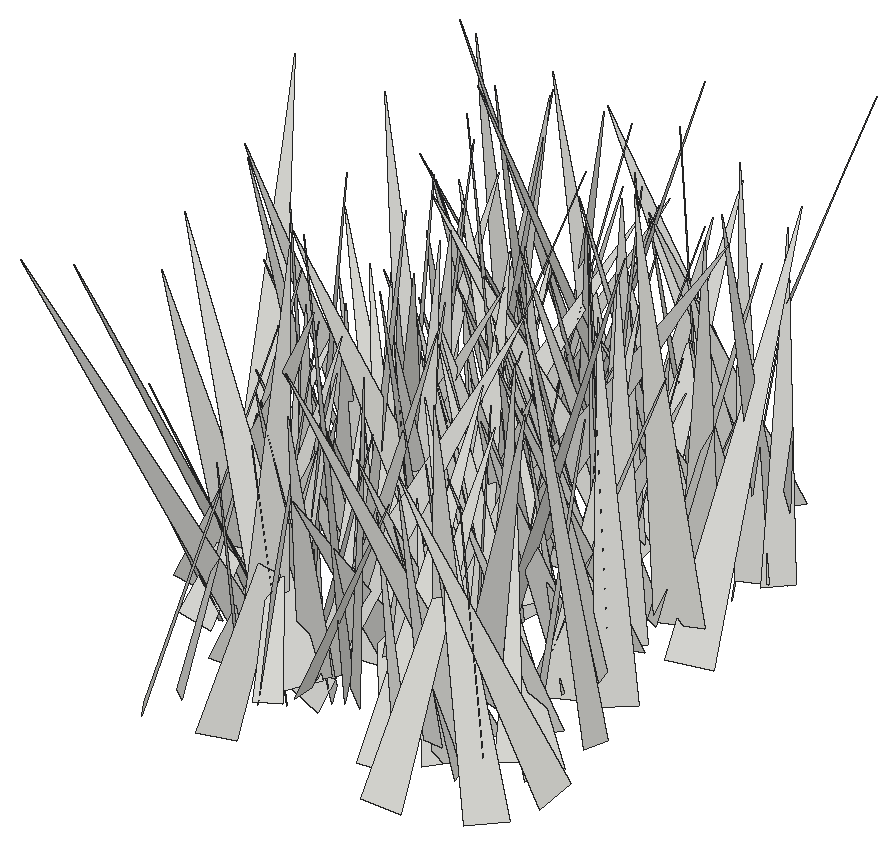
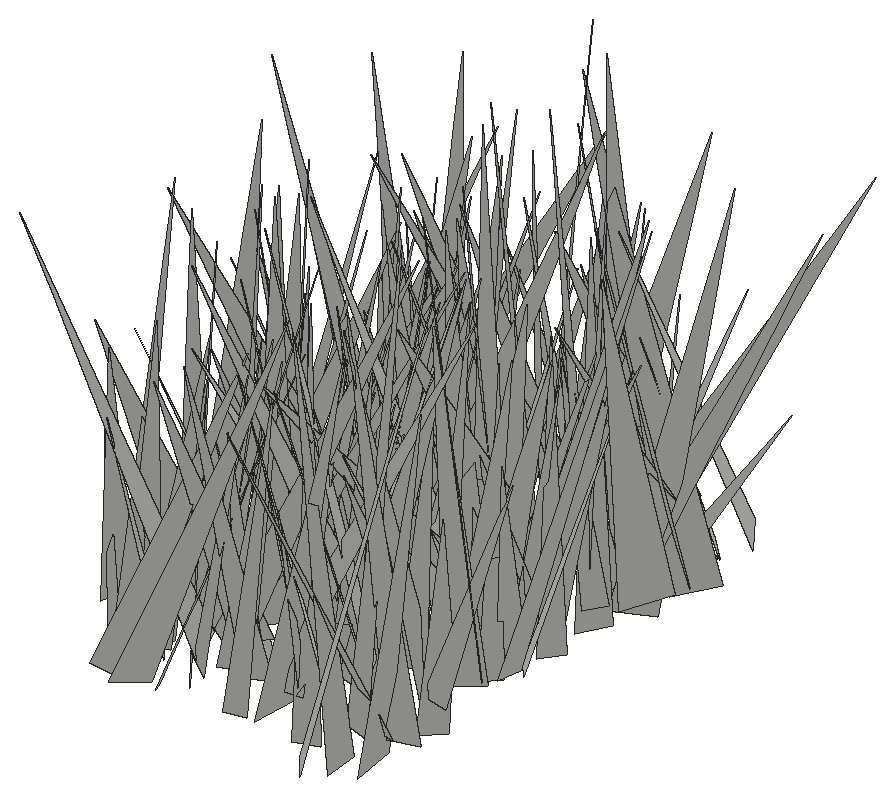
# SketchUp Ruby script. Lengths in inches.
U = 1.inch
M = Sketchup.active_model
def pt(a) = Geom::Point3d.new(a.map { |v| v * U })
def face(e, loops, mat)
  f = e.add_face(loops[0].map { |a| pt(a) })
  loops[1..].each { |l| e.add_face(l.map { |a| pt(a) }).erase! }
  f.material = f.back_material = mat if mat
  f
end
# faces: each face lists its corners as indices into pts; further lists are holes
def faces(e, pts, list, mat = nil) = list.each { |f| face(e, (f[0].is_a?(Array) ? f : [f]).map { |l| l.map { |i| pts[i] } }, mat) }
# xy, xz, yz: faces in a plane at the given z, y or x. An outline is a flat list of corners, or four numbers for a rectangle; further outlines are holes
def ring(l) = l.size == 4 ? [[l[0], l[1]], [l[2], l[1]], [l[2], l[3]], [l[0], l[3]]] : l.each_slice(2).to_a
def flat(e, list, mat, &to3) = list.each { |f| face(e, (f[0].is_a?(Array) ? f : [f]).map { |l| ring(l).map { |u, v| to3.(u, v) } }, mat) }
def xy(e, z, list, mat = nil) = flat(e, list, mat) { |x, y| [x, y, z] }
def xz(e, y, list, mat = nil) = flat(e, list, mat) { |x, z| [x, y, z] }
def yz(e, x, list, mat = nil) = flat(e, list, mat) { |y, z| [x, y, z] }
def lines(e, pts, list) = list.each { |a, b| e.add_line(pt(pts[a]), pt(pts[b])) }
# prism: a flat outline (further loops are holes) pulled along v
def prism(e, loops, v, mat = nil)
  f = face(e, loops, mat); d = Geom::Vector3d.new(v.map { |x| x * U })
  f.pushpull(f.normal.samedirection?(d) ? d.length : -d.length)
end
def box(e, o, s, mat = nil) = prism(e, [[o, [o[0] + s[0], o[1], o[2]], [o[0] + s[0], o[1] + s[1], o[2]], [o[0], o[1] + s[1], o[2]]]], [0, 0, s[2]], mat)
def at(x, y, z, deg = 0) = Geom::Transformation.translation(pt([x, y, z])) * Geom::Transformation.rotation(ORIGIN, Z_AXIS, deg.degrees)
def axes(o, x, y, z) = Geom::Transformation.new([*x, 0, *y, 0, *z, 0, *pt(o).to_a, 1])
def part(name) = M.definitions.add(name)
# library, detail: a bought-in or finely detailed component or shape, given as its bounding box
def library(name, o, s) = part(name).tap { |d| box(d.entities, o, s) }
def detail(e, o, s) = box(e.add_group.entities, o, s)
def put(e, d, t, mat = nil) = e.add_instance(d, t).tap { |i| i.material = mat if mat }
def group(e, t, mat = nil) = e.add_group.tap { |g| g.transformation = t; g.material = mat if mat }.entities
root = M.entities
c1 = part("fur_instance\#9")
p = [[0.8125,0,1.79],[0.67,-0.02,1.48],[0,-0.11,0],[0,0.11,0]]
faces(c1.entities,p,[[0,1,2,3]])
put(root,c1,axes([65.37,132.02,-27.1],[-6.50457,4.89284,0.5628],[4.72218,6.46057,-1.59001],[1.39918,0.94188,7.98255]))
put(root,c1,axes([66.375,129.34,-27.1],[-2.80536,-2.90649,0.0794],[-2.63209,2.49174,-1.78533],[-1.23535,1.29136,3.62358]))
put(root,c1,axes([67.03,130.54,-27.1],[-2.83632,-6.0499,0.28173],[-5.90232,2.69141,-1.62612],[-1.35766,0.93829,6.48088]))
put(root,c1,axes([65.68,137.62,-27.1],[-3.97352,-3.33663,0.47318],[-3.25036,3.98768,0.8243],[0.89005,-0.33346,5.12275]))
put(root,c1,axes([65.8125,138.13,-27.1],[-7.05336,-2.15617,1.71578],[-1.62887,7.06566,2.18314],[2.22256,-1.66441,7.04506]))
put(root,c1,axes([66.8,143.5,-28.22],[-7.05246,-0.20222,1.59365],[-0.38202,7.18084,-0.77939],[1.56034,0.84409,7.01218]))
put(root,c1,axes([68.76,129.2,-28.22],[-1.39061,-8.04384,0.83594],[-7.45661,0.94696,-3.29214],[-3.13068,1.31752,7.46987]))
put(root,c1,axes([66.67,136.97,-27.1],[-4.24883,1.88722,0.42776],[1.75815,4.19597,-1.04876],[0.80838,0.79335,4.52927]))
put(root,c1,axes([66.56,140.84,-27.1],[-0.08918,-3.86635,0.81214],[-3.84672,-0.10019,-0.89937],[-0.90053,0.81086,3.76135]))
put(root,c1,axes([66.54,131.21,-28.22],[4.91943,-4.73173,2.30235],[-4.40019,-5.42749,-1.75256],[-2.8859,0.2095,6.59686]))
put(root,c1,axes([68.17,136.98,-27.1],[-6.64184,2.29308,0.28161],[2.23011,6.58737,-1.04152],[0.60342,0.8944,6.94892]))
put(root,c1,axes([66.06,136.18,-27.1],[1.11267,-4.69864,0.20362],[-4.67497,-1.12782,-0.47895],[-0.51316,0.0867,4.80478]))
put(root,c1,axes([67.26,146.49,-27.1],[-6.10704,-5.17922,1.29191],[-4.99805,6.23748,1.37932],[1.87424,-0.24245,7.88782]))
put(root,c1,axes([67.74,130.69,-28.22],[-3.26059,-4.43586,0.10579],[-4.43536,3.26207,0.0775],[0.12511,0.03932,5.50476]))
put(root,c1,axes([65.54,136.41,-27.1],[4.72712,-1.54603,0.79765],[-1.39638,-4.74943,-0.93014],[-1.03759,-0.65178,4.88576]))
put(root,c1,axes([65.35,130.17,-27.1],[3.97347,4.57155,1.31094],[4.73936,-3.94824,-0.59665],[-0.39506,-1.38509,6.02757]))
put(root,c1,axes([68.65,133.42,-28.22],[-2.69995,-7.06667,2.40673],[-7.39529,2.18224,-1.88876],[-1.01973,2.88442,7.32531]))
put(root,c1,axes([65.8,128.78,-27.1],[-0.63862,5.35473,0.03552],[5.1577,0.62471,-1.44573],[1.43964,0.13724,5.19527]))
put(root,c1,axes([68.1875,134.67,-28.22],[-5.31115,0.249,1.00047],[0.14264,5.37711,-0.58108],[1.02108,0.54405,5.28514]))
put(root,c1,axes([67.35,132.58,-27.1],[-4.34525,-4.69158,2.51984],[-5.05188,4.66036,-0.03462],[1.68493,1.87398,6.3946]))
put(root,c1,axes([66.07,138.71,-27.1],[4.73789,-1.18845,0.72275],[-0.9672,-4.65874,-1.32025],[-0.99966,-1.12521,4.70287]))
put(root,c1,axes([69.15,134.625,-27.1],[-3.00084,5.06154,0.45444],[5.0055,2.85272,1.2797],[-0.87785,-1.03611,5.74339]))
put(root,c1,axes([65.71,143.39,-27.1],[-0.42435,-6.57592,2.54627],[-6.78158,1.0798,1.65847],[1.93298,2.34469,6.37748]))
put(root,c1,axes([67.03,126.5,-28.22],[3.04107,3.48011,0.59696],[3.3547,-3.09349,0.94446],[-1.10161,0.1866,4.52408]))
put(root,c1,axes([66.43,139.42,-27.1],[2.75053,-5.09352,1.52718],[-5.31748,-2.64324,0.76119],[-0.02665,1.70616,5.73847]))
put(root,c1,axes([68.98,133.01,-27.1],[-0.44719,-4.16584,0.88919],[-4.01944,0.11666,-1.47491],[-1.41032,0.98845,3.92158]))
put(root,c1,axes([66.71,125.11,-28.22],[5.18703,3.91751,0.7095],[3.72248,-5.18551,1.41748],[-1.41191,0.72053,6.34373]))
put(root,c1,axes([66.6,140.875,-28.22],[6.40589,-1.32849,1.4611],[-0.83624,-6.31798,-2.07823],[-1.78897,-1.80373,6.20333]))
put(root,c1,axes([66.84,132.75,-28.22],[5.79339,-2.08626,1.56673],[-1.97661,-6.00002,-0.68061],[-1.70297,-0.13319,6.11985]))
put(root,c1,axes([66.38,133.23,-27.1],[3.1539,-2.32332,0.00557],[-2.32207,-3.15188,0.13648],[0.07647,0.11319,3.91488]))
put(root,c1,axes([68.6,134.68,-27.1],[-1.93771,-4.14246,0.35212],[-4.15628,1.93921,-0.05843],[0.0961,0.34375,4.57288]))
put(root,c1,axes([67.24,143.76,-27.1],[-3.46246,-6.72611,1.90114],[-6.59046,3.84836,1.61233],[2.32826,0.89059,7.39118]))
put(root,c1,axes([67.82,130.51,-28.22],[0.58745,4.61701,1.14714],[4.75417,-0.52722,-0.31264],[0.17496,-1.17604,4.64372]))
put(root,c1,axes([70.76,127.48,-27.1],[-6.11884,4.72961,1.11538],[4.85918,5.97068,1.339],[0.0418,-1.7422,7.61686]))
put(root,c1,axes([68.25,138.9375,-28.22],[6.51752,3.06728,2.32468],[2.5593,-6.86862,1.88745],[-2.87443,0.8392,6.95153]))
put(root,c1,axes([68.92,128.92,-27.1],[-4.7564,-0.43454,1.78324],[-0.95829,4.81251,-1.3833],[1.56539,1.62573,4.5715]))
put(root,c1,axes([64.67,130.49,-27.1],[3.10816,-7.62871,0.22312],[-7.12075,-2.81203,3.04879],[2.74626,1.34273,7.65263]))
put(root,c1,axes([68.53,127.69,-28.22],[-2.76326,-3.0585,1.38467],[-3.15346,2.97986,0.28892],[1.15213,0.82059,4.11176]))
put(root,c1,axes([67.52,132.16,-27.1],[6.90611,3.10223,2.59996],[3.46907,-7.18559,-0.64093],[-2.08547,-1.6797,7.5437]))
put(root,c1,axes([67.55,144.13,-28.22],[6.8953,0.9557,1.85973],[1.13553,-7.09282,-0.56526],[-1.75571,-0.83402,6.93822]))
put(root,c1,axes([68.43,139.6,-27.1],[3.6116,-2.54944,1.03868],[-2.46348,-3.75778,-0.65768],[-1.22872,0.0404,4.37159]))
put(root,c1,axes([67.95,136.85,-28.22],[5.70767,4.90783,2.44546],[5.23724,-5.92496,-0.33273],[-1.62433,-1.85811,7.52021]))
put(root,c1,axes([68.91,138.86,-27.1],[-2.94733,3.27814,0.42411],[3.06608,2.92358,-1.29021],[1.23501,0.56503,4.21525]))
put(root,c1,axes([66.34,143.4,-27.1],[3.26284,4.45559,0.15103],[4.26787,-3.06768,-1.7017],[1.28856,-1.1217,5.25381]))
put(root,c1,axes([69.94,128.25,-27.1],[0.78619,5.10987,0.99795],[4.99569,-1.02461,1.31074],[-1.46621,-0.75112,5.00108]))
put(root,c1,axes([69.73,130.56,-28.22],[-3.33951,2.40161,0.05247],[2.31618,3.24301,-1.02031],[0.63702,0.79874,3.98485]))
put(root,c1,axes([66.95,128.88,-28.22],[2.87453,-4.20489,0.68169],[-4.14129,-2.56592,1.63539],[0.99777,1.46412,4.82385]))
put(root,c1,axes([71.49,142.23,-27.1],[-3.69679,-5.87263,0.02895],[-5.78236,3.6339,-1.23044],[-1.02613,0.67962,6.82936]))
put(root,c1,axes([69.74,131.6,-28.22],[-6.65412,4.03174,0.74119],[3.28122,6.08544,-3.64454],[2.45722,2.79179,6.87384]))
put(root,c1,axes([70.47,139.96,-28.22],[-0.74223,-7.02206,1.66779],[-7.14663,0.48084,-1.156],[-1.00829,1.76103,6.96591]))
put(root,c1,axes([71.25,142.75,-28.22],[-7.31689,1.04904,1.18508],[0.99417,7.40794,-0.41938],[1.23147,0.25252,7.3798]))
put(root,c1,axes([69.88,138.13,-27.1],[-4.44345,-1.97155,1.25823],[-1.71315,4.58269,1.13072],[1.59225,-0.57131,4.72787]))
put(root,c1,axes([69.67,137.2,-27.1],[3.36886,3.17868,0.5186],[2.75759,-3.23451,1.91201],[-1.66392,1.0752,4.2187]))
put(root,c1,axes([66.53,135.41,-27.1],[3.98085,5.13777,1.04709],[4.9615,-3.26572,-2.83883],[1.69606,-2.50573,5.84679]))
put(root,c1,axes([68.85,134.28,-27.1],[-0.53064,3.51066,0.60828],[3.36851,0.69471,-1.0709],[1.16098,-0.41106,3.38519]))
put(root,c1,axes([68.83,136.25,-27.1],[3.92094,-4.8226,1.73149],[-5.06492,-3.97791,0.39007],[-0.77596,1.59628,6.20315]))
put(root,c1,axes([70.7,129.43,-28.22],[-4.42725,-2.60663,1.07476],[-2.66002,4.52485,0.01676],[0.93485,0.53053,5.13759]))
put(root,c1,axes([69.54,133.97,-27.1],[4.78863,4.89843,2.46119],[5.13986,-5.14824,0.24599],[-1.90629,-1.57608,6.84581]))
put(root,c1,axes([69.38,131.54,-28.22],[3.15596,1.30372,1.61225],[1.82364,-3.14251,-1.02861],[-0.98659,-1.6383,3.25603]))
put(root,c1,axes([70.67,126.23,-27.1],[-2.92778,3.00983,0.00711],[2.98882,2.90849,-0.48849],[0.35507,0.33555,4.17041]))
put(root,c1,axes([71.4,139.18,-27.1],[-5.49942,-3.45806,0.94275],[-3.51329,5.5426,-0.16378],[0.70973,0.64178,6.49422]))
put(root,c1,axes([68.85,141.13,-27.1],[3.76051,3.97563,0.83952],[4.01253,-3.81366,0.08642],[-0.64034,-0.54974,5.47171]))
put(root,c1,axes([69.52,125.2,-28.22],[-5.19171,3.73852,1.55221],[3.028,5.26206,-2.54592],[2.68647,1.29382,5.8693]))
put(root,c1,axes([69.41,128.65,-28.22],[-3.39488,-3.98848,1.56761],[-3.7052,3.73666,1.48306],[2.15333,0.14147,5.02331]))
put(root,c1,axes([69.49,127.43,-27.1],[6.01123,-4.10409,2.83515],[-4.50522,-6.3728,0.32708],[-2.14119,1.8869,7.27128]))
put(root,c1,axes([70.33,129.08,-27.1],[-1.26664,-5.03308,1.07763],[-5.14261,1.28411,-0.04714],[0.2163,1.05675,5.1898]))
put(root,c1,axes([70.22,142.47,-28.22],[-3.5127,-1.06556,1.8883],[-1.54789,3.74984,-0.76344],[1.51826,1.35772,3.59049]))
put(root,c1,axes([72.42,130.5625,-28.22],[-2.20757,6.36235,0.08993],[6.1827,2.12231,1.62203],[-1.50393,-0.61421,6.5362]))
put(root,c1,axes([67.71,136.62,-27.1],[7.63705,-2.12328,0.08153],[-2.0044,-7.29978,-2.35267],[-0.70524,-2.24596,7.56953]))
put(root,c1,axes([68.76,135.3,-27.1],[-3.50989,5.55769,0.51718],[4.45011,3.15505,-3.70364],[3.36927,1.62248,5.4305]))
put(root,c1,axes([68.47,143.35,-27.1],[4.49917,3.28934,0.87918],[3.40387,-4.3112,-1.28935],[0.07989,-1.55853,5.42216]))
put(root,c1,axes([70.88,139.84,-28.22],[-0.51846,-5.08764,2.15235],[-5.51728,0.36879,-0.45728],[-0.27624,2.18298,5.0935]))
put(root,c1,axes([68.67,137.51,-27.1],[4.5818,0.64032,0.1617],[0.65902,-4.5067,-0.82732],[-0.04299,-0.84188,4.55176]))
put(root,c1,axes([69.31,132.33,-27.1],[-4.14785,-5.45032,3.6874],[-5.74845,5.12259,1.10541],[3.20285,2.13555,6.75935]))
put(root,c1,axes([70.46,137.42,-27.1],[2.53184,-2.74895,1.13947],[-2.76231,-2.72751,-0.44237],[-1.1067,0.51894,3.71097]))
put(root,c1,axes([70.06,126.49,-27.1],[-4.21577,-3.58718,3.5566],[-4.31781,4.96325,-0.11214],[2.62178,2.40587,5.53425]))
put(root,c1,axes([73.57,142.16,-27.1],[-3.74944,-6.99723,1.04952],[-6.92154,3.38084,-2.18706],[-1.468,1.93125,7.63127]))
put(root,c1,axes([73.15,136.16,-27.1],[-5.62336,3.63446,0.06059],[3.63174,5.6129,0.37548],[-0.15301,-0.3482,6.6851]))
put(root,c1,axes([72.71,134.41,-28.22],[-7.92224,1.63819,2.17065],[2.33717,7.51957,2.85498],[1.39032,-3.306,7.56932]))
put(root,c1,axes([68.15,136.14,-28.22],[7.55875,3.30018,0.58934],[3.3113,-7.57673,-0.04195],[-0.52327,-0.27436,8.24768]))
put(root,c1,axes([69.23,143.73,-28.22],[-1.15928,-6.64992,1.1524],[-6.36185,1.46707,2.06591],[2.25307,0.72087,6.42631]))
put(root,c1,axes([70.2,143.13,-27.1],[-1.799,-4.93024,0.4482],[-4.7112,1.85147,1.45641],[1.52075,-0.09654,5.04207]))
put(root,c1,axes([71.27,140.54,-28.22],[-1.29873,-6.18935,0.13887],[-6.18983,1.30082,0.08883],[0.11547,0.11765,6.32352]))
put(root,c1,axes([73.58,134.8,-27.1],[-7.24108,-2.76695,1.69952],[-3.23599,6.49389,-3.21487],[0.2698,3.62643,7.05364]))
put(root,c1,axes([71.74,132.01,-28.22],[-3.79874,-3.55526,0.6962],[-3.51199,3.8615,0.55657],[0.88909,0.06302,5.17306]))
put(root,c1,axes([69.42,140.1875,-27.1],[6.44327,3.68852,1.42181],[3.82977,-6.4983,-0.49739],[-0.97955,-1.14429,7.40767]))
put(root,c1,axes([71.69,139.45,-27.1],[0.72019,-3.80208,0.86926],[-3.795,-0.88705,-0.73566],[-0.89965,0.69817,3.79912]))
put(root,c1,axes([72.33,135.72,-27.1],[-0.0394,4.36961,1.02441],[4.32756,-0.23455,1.1669],[-1.18959,-0.99797,4.2111]))
put(root,c1,axes([70.69,128.61,-27.1],[1.15457,-5.41906,0.82486],[-5.48032,-1.12384,0.28761],[0.11275,0.86626,5.53322]))
put(root,c1,axes([71.11,141.57,-27.1],[3.02903,2.92229,1.12241],[2.89072,-3.2105,0.55771],[-1.2014,-0.35704,4.17178]))
put(root,c1,axes([74.0625,140.01,-27.1],[-7.08449,-0.21202,0.14595],[-0.16992,6.87165,1.73429],[0.19334,-1.72965,6.8722]))
put(root,c1,axes([72.39,137.11,-28.22],[-5.0365,1.95588,2.0654],[2.56555,4.93734,1.5806],[1.22852,-2.29236,5.16658]))
put(root,c1,axes([71.88,130.98,-27.1],[4.93577,0.48548,2.66433],[-0.37318,-5.36398,1.66873],[-2.68236,1.63958,4.67042]))
put(root,c1,axes([70.81,145.22,-27.1],[-0.56005,-4.94681,0.27227],[-4.82604,0.60667,1.09544],[1.12,0.14049,4.85639]))
put(root,c1,axes([72,128.49,-27.1],[-6.4664,-4.252,2.80304],[-4.40658,6.94256,0.3657],[2.55316,1.21333,7.73047]))
put(root,c1,axes([71.24,132.29,-28.22],[4.70734,-3.12135,0.14145],[-2.64852,-4.12178,-2.81392],[-1.65776,-2.27815,4.89732]))
put(root,c1,axes([69.96,129.47,-27.1],[5.00049,1.26706,0.71261],[1.41038,-4.84715,-1.27832],[-0.35226,-1.4205,4.99762]))
put(root,c1,axes([70.56,134.75,-28.22],[6.56004,-2.8558,0.90961],[-2.50702,-6.42798,-2.10074],[-1.6425,-1.59457,6.83935]))
put(root,c1,axes([72.13,135.86,-27.1],[-0.71572,-3.67555,0.46048],[-3.70429,0.70984,-0.09154],[-0.00255,0.46948,3.74347]))
put(root,c1,axes([72.99,130.15,-27.1],[-6.34351,2.24327,1.15963],[1.89857,6.30395,-1.80908],[1.66506,1.35834,6.48071]))
put(root,c1,axes([71.18,128.67,-27.1],[5.70541,0.17051,1.69377],[-0.31532,-5.71566,1.63753],[-1.67287,1.65887,5.46803]))
put(root,c1,axes([71.65,133.24,-28.22],[-3.5221,-6.63629,1.77015],[-6.5539,3.84233,1.36448],[2.0543,0.8804,7.38808]))
put(root,c1,axes([73.75,133.95,-28.22],[-1.46223,5.38545,2.28823],[5.73287,0.84616,1.67196],[-1.17188,-2.58033,5.32407]))
put(root,c1,axes([73.5,134.38,-28.22],[-4.56615,-2.82263,0.99228],[-2.92894,4.58662,-0.43101],[0.61084,0.89289,5.35081]))
put(root,c1,axes([72.5,133.3,-28.22],[-3.43213,5.64571,1.59286],[5.69776,3.64732,-0.65059],[1.39526,-1.00684,6.57497]))
put(root,c1,axes([70.51,135.82,-27.1],[2.89103,-3.61881,0.35286],[-3.55779,-2.72252,1.22815],[0.74997,1.03461,4.46604]))
put(root,c1,axes([71.63,138.11,-27.1],[6.96857,3.90701,1.2479],[3.36407,-6.85211,2.66731],[-2.34628,1.77954,7.53068]))
put(root,c1,axes([70.6,136.81,-28.22],[4.92318,-0.35306,0.35659],[-0.43613,-4.74982,1.31852],[-0.24819,1.34315,4.75646]))
put(root,c1,axes([74.56,145.6,-27.1],[-6.62778,2.24684,1.33683],[2.5489,6.36376,1.94128],[0.58185,-2.2841,6.72363]))
put(root,c1,axes([72.47,139.86,-28.22],[-3.28751,-5.48957,1.02333],[-5.33666,3.43821,1.29963],[1.64396,0.18343,6.2653]))
put(root,c1,axes([71.15,127.38,-27.1],[4.07736,0.20577,0.16386],[0.20057,-4.0788,0.13116],[-0.17019,0.12285,4.08044]))
put(root,c1,axes([69.88,128.74,-28.22],[0.84349,7.5995,0.98427],[7.14395,-0.42161,-2.86687],[2.77222,-1.22577,7.08837]))
put(root,c1,axes([72.26,136.79,-27.1],[3.35364,-3.87615,0.32814],[-3.76663,-3.34394,-1.00479],[-0.97195,-0.41544,5.02611]))
put(root,c1,axes([72.58,128.13,-27.1],[-3.23296,-4.09809,2.47034],[-4.47809,3.64184,0.18098],[1.68632,1.81429,5.21667]))
put(root,c1,axes([71.62,143.1,-27.1],[0.44835,5.06558,1.88586],[5.29017,-0.02286,-1.19629],[1.10933,-1.93829,4.94267]))
put(root,c1,axes([73.49,143.625,-27.1],[-2.97615,-4.05495,1.48787],[-4.26463,3.04523,-0.23114],[0.68511,1.34083,5.02461]))
put(root,c1,axes([73.92,138.73,-28.22],[-5.06877,-1.96642,0.89661],[-1.81084,5.11214,0.97466],[1.17965,-0.60192,5.34876]))
put(root,c1,axes([75.3125,139.07,-28.22],[-0.2537,5.53184,2.90433],[5.7111,-0.97344,2.35297],[-2.53371,-2.74807,5.0129]))
put(root,c1,axes([72.57,143.06,-27.1],[2.27929,-4.31761,0.37807],[-4.29346,-2.30768,-0.46977],[-0.59235,0.11282,4.85966]))
put(root,c1,axes([72.09,142.78,-27.1],[1.922,-3.18961,0.22781],[-3.1707,-1.86642,0.61867],[0.41494,0.51232,3.67219]))
put(root,c1,axes([71.81,136.74,-28.22],[4.41125,2.39111,1.26664],[2.67652,-4.21168,-1.37073],[-0.39751,-1.82353,4.82677]))
put(root,c1,axes([72.25,136.93,-27.1],[5.97611,0.87511,2.00016],[1.66713,-5.59279,-2.53411],[-1.40966,-2.90435,5.48252]))
put(root,c1,axes([73.21,141.34,-27.1],[-2.73527,5.15415,0.70761],[4.98067,2.82527,-1.3261],[1.50298,0.0175,5.68229]))
put(root,c1,axes([72.125,139.1,-28.22],[4.87544,3.99495,1.42226],[4.19795,-4.85335,-0.75795],[-0.59966,-1.4959,6.2574]))
put(root,c1,axes([72.94,140.7,-28.22],[3.50621,1.98379,0.78234],[2.0421,-3.55715,-0.13217],[-0.61424,-0.50223,4.02634]))
put(root,c1,axes([73.64,130.66,-27.1],[-2.96386,2.60362,0.59977],[2.15648,2.85999,-1.75873],[1.5774,0.98217,3.53132]))
put(root,c1,axes([74.78,141.4,-27.1],[2.18952,-4.24382,2.13551],[-4.35668,-2.73133,-0.96101],[-1.89466,1.3763,4.67766]))
put(root,c1,axes([75.78,140.87,-28.22],[-6.35383,-3.10693,1.06991],[-3.1587,6.41685,-0.12448],[0.9057,0.58302,7.07168]))
put(root,c1,axes([75.44,145.57,-27.1],[1.50286,-5.49819,1.33251],[-5.18917,-1.88889,-1.94134],[-2.25347,0.68284,5.35909]))
put(root,c1,axes([73.36,140.02,-27.1],[4.72126,-4.87179,1.88096],[-5.03873,-4.91595,-0.08523],[-1.37242,1.28908,6.78361]))
put(root,c1,axes([76.3,138.625,-27.1],[-6.09623,-2.24198,1.5344],[-2.70516,5.35755,-2.91953],[0.25098,3.28863,5.80232]))
put(root,c1,axes([74.78,130.87,-27.1],[-4.80536,-1.45342,1.08645],[-0.98448,4.67157,1.89512],[1.52434,-1.5647,4.64891]))
put(root,c1,axes([74.97,143.76,-28.22],[-4.74866,-3.13825,0.27488],[-2.86364,4.50737,1.98925],[1.31291,-1.51952,5.33303]))
put(root,c1,axes([74.14,135.64,-28.22],[5.32818,4.49942,0.50618],[3.89144,-4.95023,3.04014],[-2.31467,2.03493,6.2763]))
put(root,c1,axes([74.71,142.5,-28.22],[-5.77727,-4.35757,2.82703],[-4.73437,6.15702,-0.18467],[2.13687,1.8601,7.23403]))
put(root,c1,axes([70.34,137.48,-27.1],[5.69226,-5.26322,0.96159],[-5.00885,-4.7486,3.65927],[1.88086,3.28288,6.8347]))
put(root,c1,axes([77.17,128.71,-27.1],[-0.65869,-6.64833,1.3688],[-6.16249,0.00919,-2.92087],[-2.84565,1.51902,6.00855]))
put(root,c1,axes([76.1875,133.91,-28.22],[-4.28089,-1.18354,0.47624],[-1.27514,3.91753,-1.72642],[-0.03977,1.79046,4.09221]))
put(root,c1,axes([75.55,126.59,-27.1],[-3.65849,-0.26653,0.63033],[-0.40108,3.61269,-0.80033],[0.55452,0.85461,3.57982]))
put(root,c1,axes([74.61,126.66,-28.22],[-1.71935,6.00909,0.23442],[5.94835,1.73522,-0.85232],[0.8839,0.01135,6.19184]))
put(root,c1,axes([75.8,128,-28.22],[-3.60805,2.068,0.36238],[2.05277,3.62596,-0.25393],[0.44056,0.04128,4.15092]))
put(root,c1,axes([74.46,137.9,-28.22],[-2.53313,-4.37285,1.78451],[-4.47538,2.86942,0.67851],[1.50904,1.16947,5.00781]))
put(root,c1,axes([75.375,130.17,-28.22],[0.00503,4.167,0.7042],[4.17874,-0.11,0.62111],[-0.63075,-0.69557,4.12045]))
put(root,c1,axes([74.79,135.23,-27.1],[4.72297,-1.05883,1.70864],[-0.28791,-4.67444,-2.10088],[-1.98939,-1.83725,4.36049]))
put(root,c1,axes([75.08,139.66,-27.1],[4.55418,4.59674,3.34406],[5.23121,-5.06575,-0.16086],[-2.22422,-2.50228,6.46875]))
put(root,c1,axes([74.67,132.22,-28.22],[5.47635,-0.94494,2.24683],[-1.1073,-5.8869,0.22307],[-2.17142,0.61884,5.55279]))
put(root,c1,axes([76.64,135.11,-28.22],[-6.75602,-0.97126,1.58692],[-1.43223,6.52998,-2.10085],[1.1876,2.34979,6.49412]))
put(root,c1,axes([74.69,131.15,-28.22],[4.34542,2.75412,2.00138],[2.98226,-4.64462,-0.0836],[-1.6422,-1.14703,5.14401]))
put(root,c1,axes([75.32,143.56,-27.1],[3.57581,-3.48366,1.446],[-3.33217,-3.85124,-1.03819],[-1.76733,0.21279,4.88308]))
put(root,c1,axes([73.53,137.98,-27.1],[3.09859,-2.8989,0.71648],[-2.92503,-2.73871,1.56906],[0.60101,1.61681,3.94246]))
put(root,c1,axes([78.82,129.53,-28.22],[-1.95645,6.57203,0.15793],[5.85701,1.66776,3.15567],[-2.98529,-1.03499,6.08778]))
put(root,c1,axes([74.96,136.08,-27.1],[2.81827,1.89164,1.24112],[2.11841,-2.90244,-0.38665],[-0.79437,-1.02901,3.37216]))
put(root,c1,axes([76.8,127.81,-28.22],[-3.69691,-1.68274,0.52652],[-1.75981,3.59718,-0.85985],[0.10916,1.00233,3.96981]))
put(root,c1,axes([75.32,143.05,-27.1],[3.88583,-1.17381,1.38743],[-0.79486,-4.04284,-1.19419],[-1.63432,-0.82466,3.87962]))
put(root,c1,axes([76.19,127.37,-27.1],[-1.43157,-3.77915,1.63266],[-4.11341,1.2436,-0.72817],[-0.16553,1.78,3.97506]))
put(root,c1,axes([76.35,134.57,-28.22],[5.18637,5.57386,2.23152],[5.04396,-5.64447,2.37581],[-3.2567,0.13438,7.23339]))
put(root,c1,axes([75.72,136.45,-27.1],[4.83002,3.67653,3.08875],[4.26917,-5.29337,-0.3752],[-2.19806,-2.20219,6.05848]))
put(root,c1,axes([77.23,135.65,-27.1],[-0.62326,-5.57048,0.69706],[-5.46922,0.44429,-1.33972],[-1.26641,0.82277,5.44278]))
put(root,c1,axes([77.51,141.21,-27.1],[0.02975,6.47261,1.15989],[6.34372,-0.33363,1.69906],[-1.73125,-1.11127,6.2457]))
put(root,c1,axes([76.34,141.72,-28.22],[3.7445,3.22853,1.26331],[2.91821,-3.9391,1.41711],[-1.87174,0.31742,4.73672]))
put(root,c1,axes([76.2,133.5625,-28.22],[-4.85985,3.92503,1.53679],[3.59209,5.08366,-1.6245],[2.20555,0.36911,6.032]))
put(root,c1,axes([74.08,142.54,-27.1],[7.5502,3.19495,0.69372],[3.12341,-7.56468,0.84526],[-0.96605,0.51231,8.15468]))
put(root,c1,axes([73.93,133.5,-27.1],[7.81228,1.65656,1.00866],[1.73052,-7.84393,-0.52089],[-0.87571,-0.72239,7.96898]))
put(root,c1,axes([77.59,134.04,-27.1],[-4.87581,-1.54153,0.97742],[-1.54685,4.96967,0.12147],[0.96896,0.17664,5.11224]))
put(root,c1,axes([77.79,126.97,-27.1],[1.94279,3.86541,2.10519],[3.74501,-2.66073,1.42935],[-2.3126,-1.06149,4.08323]))
put(root,c1,axes([76.14,124.89,-28.22],[-1.14169,6.19263,0.48775],[6.13199,1.20279,-0.91762],[0.99261,-0.30768,6.22978]))
put(root,c1,axes([75.9,140.72,-27.1],[0.59547,-6.22896,1.95156],[-6.50827,-0.41619,0.65745],[0.50087,1.99748,6.22272]))
put(root,c1,axes([76.89,135.83,-27.1],[3.45962,-4.50001,2.91683],[-5.02174,-3.93643,-0.1168],[-1.88153,2.2319,5.67498]))
put(root,c1,axes([78.6,130.24,-27.1],[-1.09532,-3.977,1.33167],[-3.82769,0.38536,-1.99748],[-1.71426,1.68065,3.6092]))
put(root,c1,axes([75.18,133.48,-28.22],[4.56753,3.50086,0.36537],[3.49009,-4.58212,0.27435],[-0.45689,-0.00383,5.74831]))
put(root,c1,axes([76.29,128.39,-28.22],[2.81734,-6.20209,1.85033],[-6.41792,-2.93797,-0.07572],[-0.83667,1.65211,6.81158]))
put(root,c1,axes([76.6875,137.375,-27.1],[3.68113,4.53912,0.36663],[4.24955,-3.59341,1.82137],[-1.63686,0.87892,5.5531]))
put(root,c1,axes([77.43,137.78,-27.1],[-2.10134,6.53759,3.4605],[7.38552,2.05442,0.60354],[0.41142,-3.48856,6.84043]))
put(root,c1,axes([77.64,127.32,-27.1],[-3.40834,-0.81843,0.94444],[-0.85751,3.5273,-0.03792],[0.90911,0.25869,3.50503]))
put(root,c1,axes([77.82,134.21,-28.22],[-4.07853,4.6775,2.02917],[4.97181,4.22458,0.25488],[1.13033,-1.70436,6.20068]))
put(root,c1,axes([79.3,126.11,-28.22],[-3.01404,5.97197,0.86388],[5.95256,2.78442,1.51964],[-0.98886,-1.44144,6.51457]))
put(root,c1,axes([76.64,143.28,-27.1],[6.75782,0.35235,2.65885],[1.16075,-6.88187,-2.03823],[-2.41791,-2.31896,6.45275]))
put(root,c1,axes([78.27,141.5625,-27.1],[-5.05186,2.37101,0.85511],[2.22237,5.09377,-0.9944],[1.18912,0.55319,5.49128]))
put(root,c1,axes([77.76,127.8125,-28.22],[-1.30466,-3.28465,1.2487],[-3.51229,1.2605,-0.354],[0.10971,1.29326,3.5165]))
put(root,c1,axes([77.97,137.61,-28.22],[-5.16112,5.15909,0.10388],[4.87926,4.92701,-2.27629],[1.67923,1.54029,6.93338]))
put(root,c1,axes([75.44,130.53,-27.1],[0.87943,-6.58228,1.27772],[-6.45662,-0.48373,1.95201],[1.80858,1.47376,6.34739]))
put(root,c1,axes([80.11,130.4,-27.1],[-7.13799,-1.18277,0.6594],[-1.323,6.84565,-2.04241],[0.28881,2.12669,6.94107]))
put(root,c1,axes([77.62,130.66,-27.1],[2.96652,3.66752,1.13191],[3.55325,-3.16507,0.94281],[-1.45132,-0.25254,4.62191]))
put(root,c1,axes([77.86,127.76,-27.1],[-3.21218,-2.63282,1.4726],[-2.81239,3.39173,-0.07071],[1.09119,0.99138,4.15269]))
put(root,c1,axes([78.66,127.96,-27.1],[-2.98771,2.56269,0.00271],[2.54357,2.96592,-0.47684],[0.31249,0.36018,3.90722]))
put(root,c1,axes([76.6,143.75,-28.22],[-1.05562,-3.90874,0.84941],[-3.49411,1.32871,1.77194],[1.94702,0.26528,3.64044]))
put(root,c1,axes([79.89,128.7,-28.22],[-6.07615,0.58264,0.90457],[0.83184,5.83413,1.82981],[0.68247,-1.92372,5.8233]))
